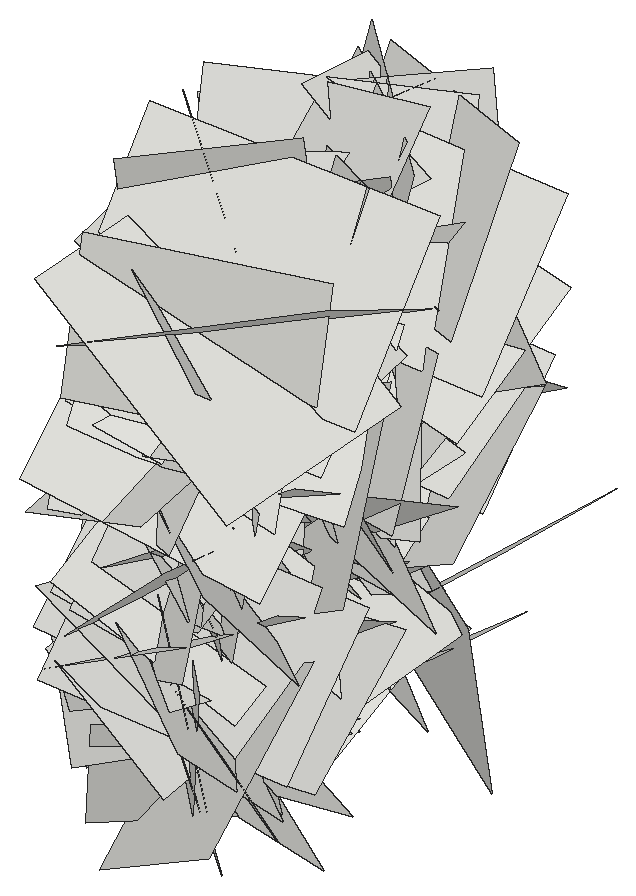
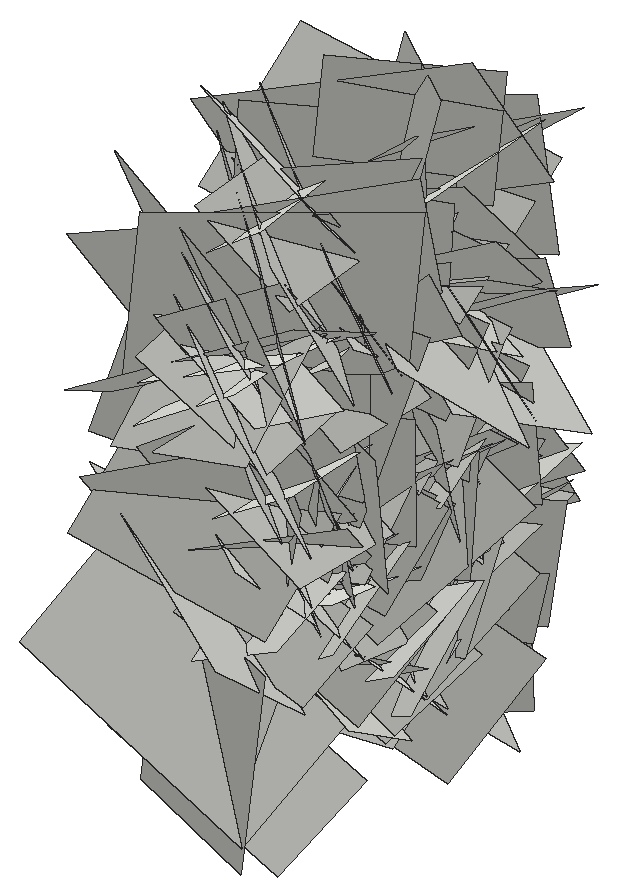
# SketchUp Ruby script. Lengths in inches.
U = 1.inch
M = Sketchup.active_model
def pt(a) = Geom::Point3d.new(a.map { |v| v * U })
def face(e, loops, mat)
  f = e.add_face(loops[0].map { |a| pt(a) })
  loops[1..].each { |l| e.add_face(l.map { |a| pt(a) }).erase! }
  f.material = f.back_material = mat if mat
  f
end
# faces: each face lists its corners as indices into pts; further lists are holes
def faces(e, pts, list, mat = nil) = list.each { |f| face(e, (f[0].is_a?(Array) ? f : [f]).map { |l| l.map { |i| pts[i] } }, mat) }
# xy, xz, yz: faces in a plane at the given z, y or x. An outline is a flat list of corners, or four numbers for a rectangle; further outlines are holes
def ring(l) = l.size == 4 ? [[l[0], l[1]], [l[2], l[1]], [l[2], l[3]], [l[0], l[3]]] : l.each_slice(2).to_a
def flat(e, list, mat, &to3) = list.each { |f| face(e, (f[0].is_a?(Array) ? f : [f]).map { |l| ring(l).map { |u, v| to3.(u, v) } }, mat) }
def xy(e, z, list, mat = nil) = flat(e, list, mat) { |x, y| [x, y, z] }
def xz(e, y, list, mat = nil) = flat(e, list, mat) { |x, z| [x, y, z] }
def yz(e, x, list, mat = nil) = flat(e, list, mat) { |y, z| [x, y, z] }
def lines(e, pts, list) = list.each { |a, b| e.add_line(pt(pts[a]), pt(pts[b])) }
# prism: a flat outline (further loops are holes) pulled along v
def prism(e, loops, v, mat = nil)
  f = face(e, loops, mat); d = Geom::Vector3d.new(v.map { |x| x * U })
  f.pushpull(f.normal.samedirection?(d) ? d.length : -d.length)
end
def box(e, o, s, mat = nil) = prism(e, [[o, [o[0] + s[0], o[1], o[2]], [o[0] + s[0], o[1] + s[1], o[2]], [o[0], o[1] + s[1], o[2]]]], [0, 0, s[2]], mat)
def at(x, y, z, deg = 0) = Geom::Transformation.translation(pt([x, y, z])) * Geom::Transformation.rotation(ORIGIN, Z_AXIS, deg.degrees)
def axes(o, x, y, z) = Geom::Transformation.new([*x, 0, *y, 0, *z, 0, *pt(o).to_a, 1])
def part(name) = M.definitions.add(name)
# library, detail: a bought-in or finely detailed component or shape, given as its bounding box
def library(name, o, s) = part(name).tap { |d| box(d.entities, o, s) }
def detail(e, o, s) = box(e.add_group.entities, o, s)
def put(e, d, t, mat = nil) = e.add_instance(d, t).tap { |i| i.material = mat if mat }
def group(e, t, mat = nil) = e.add_group.tap { |g| g.transformation = t; g.material = mat if mat }.entities
root = M.entities
c1 = part("Component\#6")
p = [[0.01,0,0],[0,3.24,4.54],[4.32,3.24,4.54],[4.33,0,0]]
faces(c1.entities,p,[[0,1,2,3]])
put(root,c1,axes([420.52,168.24,29.62],[-0.00844,-0.1319,-0.59476],[-0.00779,-0.59475,0.132],[0.64572,-0.0089,-0.00618]))
put(root,c1,axes([420.52,163.79,31.02],[-0.0186,-0.39942,0.51021],[-0.04828,0.50989,0.39761],[0.68514,0.02509,0.04187]))
put(root,c1,axes([420.52,167.3,30.05],[-0.09755,-0.36279,0.79394],[-0.2327,0.7823,0.33203],[0.89554,0.16375,0.17276]))
put(root,c1,axes([420.52,166.74,28.03],[-0.20581,0.5378,0.53941],[0.0447,0.5634,-0.54654],[0.80617,0.10606,0.16802]))
put(root,c1,axes([420.52,165.16,26.22],[0.00662,-0.41647,0.48084],[-0.04981,0.47925,0.41571],[0.67246,0.0396,0.02606]))
put(root,c1,axes([424.49,162.15,25.43],[0.09766,0.84172,-0.54191],[-0.18116,-0.52299,-0.84139],[-1.04557,0.16923,0.09516]))
put(root,c1,axes([420.52,170.38,37.22],[-0.01844,-0.65259,0.06973],[-0.0154,0.07012,0.65262],[0.69551,-0.01575,0.0163]))
put(root,c1,axes([424.49,159.15,32.85],[0.28722,0.93511,0.86971],[0.00467,0.88838,-0.95656],[-1.35365,0.20148,0.18123]))
put(root,c1,axes([420.52,168.23,31.98],[-0.11552,-0.73847,0.10601],[0.00435,0.10653,0.74638],[0.79079,-0.10846,0.01138]))
put(root,c1,axes([420.52,162.33,29.83],[-0.22776,0.38392,-0.75072],[0.01782,-0.77261,-0.39993],[0.89361,0.11326,-0.18337]))
put(root,c1,axes([424.49,165.04,27.71],[0.04822,0.07219,0.94774],[-0.14201,0.93984,-0.06516],[-0.99746,-0.13032,0.05509]))
put(root,c1,axes([420.52,171.91,32.4],[0.07209,-0.36069,-0.54144],[-0.07785,-0.54516,0.35394],[0.6852,-0.024,0.09718]))
put(root,c1,axes([424.49,167.29,35.58],[-0.17595,-0.29467,-0.74084],[-0.05215,-0.7515,0.30993],[-0.84352,0.10793,0.13537]))
put(root,c1,axes([424.49,157.3125,32.29],[0.25179,1.05256,0.51222],[-0.06429,0.53303,-1.06718],[-1.23914,0.18623,0.15945]))
put(root,c1,axes([420.52,168.82,35.84],[0.04533,0.37689,0.51175],[-0.01637,0.51337,-0.3768],[0.67349,-0.01289,-0.04361]))
put(root,c1,axes([420.52,159.46,22.85],[-0.09982,-0.0635,0.89488],[-0.1784,0.88507,0.04509],[0.93408,0.16225,0.10424]))
put(root,c1,axes([420.52,160.06,22.6],[-0.02839,-0.24478,0.77995],[-0.15528,0.76918,0.23637],[0.85248,0.13195,0.06903]))
put(root,c1,axes([420.52,159.67,28.14],[-0.12868,0.67272,0.52517],[-0.08613,0.51893,-0.68352],[0.90053,0.14576,0.00967]))
put(root,c1,axes([424.49,167.34,31.77],[0.2501,0.51374,1.1242],[0.05799,1.13903,-0.532],[-1.3089,0.14863,0.19123]))
put(root,c1,axes([420.52,158.39,26.84],[-0.02686,0.84806,0.10272],[-0.17857,0.09579,-0.83237],[0.88773,0.04493,-0.16432]))
put(root,c1,axes([420.52,169.17,27.35],[0.00515,-0.4485,-0.48712],[0.04455,-0.48594,0.44784],[0.70046,0.0342,-0.02491]))
put(root,c1,axes([424.49,161.79,25.53],[-0.01152,-0.82607,0.19056],[-0.15176,0.18963,0.81386],[-0.88572,-0.02175,-0.14193]))
put(root,c1,axes([424.49,164.2,31.01],[0.06613,-0.18181,-0.96198],[-0.02897,-0.96387,0.1804],[-1.03734,0.01533,-0.06637]))
put(root,c1,axes([420.52,169.92,30.86],[0.08798,0.07784,-0.70174],[-0.08853,-0.70052,-0.08758],[0.74315,-0.09267,0.07264]))
put(root,c1,axes([424.49,162.32,28.44],[-0.12821,-0.42216,-0.69512],[0.01339,-0.70366,0.42514],[-0.86197,0.05186,0.11]))
put(root,c1,axes([424.49,166.33,22.3],[0.05809,-0.87115,0.26873],[-0.09257,0.26296,0.87026],[-0.96191,-0.07791,-0.06752]))
put(root,c1,axes([424.49,171.77,39.47],[0.25632,-0.1505,-1.28885],[0.2021,-1.29268,0.18672],[-1.36053,-0.22038,-0.21508]))
put(root,c1,axes([420.52,167.69,34.89],[0.01272,-0.59445,-0.3878],[0.01652,-0.38754,0.59453],[0.75216,0.01856,-0.0065]))
put(root,c1,axes([420.52,168.18,25.35],[0.0356,-0.79141,-0.13903],[-0.13499,-0.14264,0.78117],[0.84098,0.01061,0.13127]))
put(root,c1,axes([424.49,163.85,33.45],[0.03445,-0.73428,-0.4148],[-0.17499,-0.41262,0.71747],[-0.87664,0.05351,-0.15952]))
put(root,c1,axes([424.49,158.45,30.92],[0.16236,0.46297,0.88251],[-0.09478,0.89566,-0.45434],[-1.05211,-0.00924,0.17712]))
put(root,c1,axes([424.49,166.53,31.68],[0.02185,0.89564,-0.0065],[-0.05171,-0.00537,-0.89456],[-0.948,0.02094,0.04865]))
put(root,c1,axes([424.49,171.21,38.93],[0.24063,-0.51313,-1.11059],[0.16085,-1.10901,0.54342],[-1.28679,-0.23458,-0.13976]))
put(root,c1,axes([420.52,171.89,34.33],[-0.10287,-0.74562,-0.1631],[0.15609,-0.17961,0.73351],[0.79385,-0.06131,-0.16536]))
put(root,c1,axes([424.49,162.43,26.35],[-0.02315,-0.70596,0.51236],[0.01203,0.51225,0.70629],[-0.92456,0.02434,-0.00364]))
put(root,c1,axes([424.49,162.61,28.57],[0.04222,-0.49534,0.62953],[-0.20196,0.60636,0.48917],[-0.82474,-0.17384,-0.08755]))
put(root,c1,axes([424.49,162.92,24.26],[-0.16568,0.16434,-0.80239],[0.1251,-0.80382,-0.18763],[-0.85913,-0.14874,0.12742]))
put(root,c1,axes([424.49,164.5,23.79],[-0.04443,0.667,0.37408],[-0.11412,0.36576,-0.66423],[-0.80255,-0.08894,0.07374]))
put(root,c1,axes([424.49,168.875,35.8],[-0.07444,0.7996,-0.0855],[-0.00091,-0.0859,-0.80263],[-0.85241,-0.06974,0.00832]))
put(root,c1,axes([420.52,164.96,33.58],[0.03363,-0.67551,-0.53197],[-0.14584,-0.52946,0.66412],[0.89967,-0.06058,0.12754]))
put(root,c1,axes([420.52,169.82,24.93],[0.00586,-0.68753,0.27068],[0.05817,0.27032,0.6855],[0.78107,-0.01497,-0.05308]))
put(root,c1,axes([424.49,164.8,26.41],[-0.06555,-0.88967,-0.10275],[0.1194,-0.1099,0.88381],[-0.94178,0.04799,0.1192]))
put(root,c1,axes([424.49,163.99,40.83],[-0.08038,0.23372,-0.81219],[0.10222,-0.80774,-0.24144],[-0.89001,-0.11388,0.04562]))
put(root,c1,axes([424.49,167.51,23.32],[0.04127,-0.8056,0.43064],[0.05085,0.43224,0.80425],[-0.96695,-0.01165,0.06068]))
put(root,c1,axes([424.49,164.95,29.96],[0.04265,0.57286,-0.52342],[-0.15347,-0.50938,-0.56862],[-0.80809,0.12697,0.08036]))
put(root,c1,axes([420.52,164.95,29.96],[-0.04265,0.57286,-0.52342],[0.15347,-0.50938,-0.56862],[0.80809,0.12697,0.08036]))
put(root,c1,axes([420.52,167.51,23.32],[-0.04127,-0.8056,0.43064],[-0.05085,0.43224,0.80425],[0.96695,-0.01165,0.06068]))
put(root,c1,axes([420.52,163.99,40.83],[0.08038,0.23372,-0.81219],[-0.10222,-0.80774,-0.24144],[0.89001,-0.11388,0.04562]))
put(root,c1,axes([420.52,164.8,26.41],[0.06555,-0.88967,-0.10275],[-0.1194,-0.1099,0.88381],[0.94178,0.04799,0.1192]))
put(root,c1,axes([424.49,169.82,24.93],[-0.00586,-0.68753,0.27068],[-0.05817,0.27032,0.6855],[-0.78107,-0.01497,-0.05308]))
put(root,c1,axes([424.49,164.96,33.58],[-0.03363,-0.67551,-0.53197],[0.14584,-0.52946,0.66412],[-0.89967,-0.06058,0.12754]))
put(root,c1,axes([420.52,168.875,35.8],[0.07444,0.7996,-0.0855],[0.00091,-0.0859,-0.80263],[0.85241,-0.06974,0.00832]))
put(root,c1,axes([420.52,164.5,23.79],[0.04443,0.667,0.37408],[0.11412,0.36576,-0.66423],[0.80255,-0.08894,0.07374]))
put(root,c1,axes([420.52,162.92,24.26],[0.16568,0.16434,-0.80239],[-0.1251,-0.80382,-0.18763],[0.85913,-0.14874,0.12742]))
put(root,c1,axes([420.52,162.61,28.57],[-0.04222,-0.49534,0.62953],[0.20196,0.60636,0.48917],[0.82474,-0.17384,-0.08755]))
put(root,c1,axes([420.52,162.43,26.35],[0.02315,-0.70596,0.51236],[-0.01203,0.51225,0.70629],[0.92456,0.02434,-0.00364]))
put(root,c1,axes([424.49,171.89,34.33],[0.10287,-0.74562,-0.1631],[-0.15609,-0.17961,0.73351],[-0.79385,-0.06131,-0.16536]))
put(root,c1,axes([420.52,171.21,38.93],[-0.24063,-0.51313,-1.11059],[-0.16085,-1.10901,0.54342],[1.28679,-0.23458,-0.13976]))
put(root,c1,axes([420.52,166.53,31.68],[-0.02185,0.89564,-0.0065],[0.05171,-0.00537,-0.89456],[0.948,0.02094,0.04865]))
put(root,c1,axes([420.52,158.45,30.92],[-0.16236,0.46297,0.88251],[0.09478,0.89566,-0.45434],[1.05211,-0.00924,0.17712]))
put(root,c1,axes([420.52,163.85,33.45],[-0.03445,-0.73428,-0.4148],[0.17499,-0.41262,0.71747],[0.87664,0.05351,-0.15952]))
put(root,c1,axes([424.49,168.18,25.35],[-0.0356,-0.79141,-0.13903],[0.13499,-0.14264,0.78117],[-0.84098,0.01061,0.13127]))
put(root,c1,axes([424.49,167.69,34.89],[-0.01272,-0.59445,-0.3878],[-0.01652,-0.38754,0.59453],[-0.75216,0.01856,-0.0065]))
put(root,c1,axes([420.52,171.77,39.47],[-0.25632,-0.1505,-1.28885],[-0.2021,-1.29268,0.18672],[1.36053,-0.22038,-0.21508]))
put(root,c1,axes([420.52,166.33,22.3],[-0.05809,-0.87115,0.26873],[0.09257,0.26296,0.87026],[0.96191,-0.07791,-0.06752]))
put(root,c1,axes([420.52,162.32,28.44],[0.12821,-0.42216,-0.69512],[-0.01339,-0.70366,0.42514],[0.86197,0.05186,0.11]))
put(root,c1,axes([424.49,169.92,30.86],[-0.08798,0.07784,-0.70174],[0.08853,-0.70052,-0.08758],[-0.74315,-0.09267,0.07264]))
put(root,c1,axes([420.52,164.2,31.01],[-0.06613,-0.18181,-0.96198],[0.02897,-0.96387,0.1804],[1.03734,0.01533,-0.06637]))
put(root,c1,axes([420.52,161.79,25.53],[0.01152,-0.82607,0.19056],[0.15176,0.18963,0.81386],[0.88572,-0.02175,-0.14193]))
put(root,c1,axes([424.49,169.17,27.35],[-0.00515,-0.4485,-0.48712],[-0.04455,-0.48594,0.44784],[-0.70046,0.0342,-0.02491]))
put(root,c1,axes([424.49,158.39,26.84],[0.02686,0.84806,0.10272],[0.17857,0.09579,-0.83237],[-0.88773,0.04493,-0.16432]))
put(root,c1,axes([424.49,159.67,28.14],[0.12868,0.67272,0.52517],[0.08613,0.51893,-0.68352],[-0.90053,0.14576,0.00967]))
put(root,c1,axes([424.49,160.06,22.6],[0.02839,-0.24478,0.77995],[0.15528,0.76918,0.23637],[-0.85248,0.13195,0.06903]))
put(root,c1,axes([424.49,159.46,22.85],[0.09982,-0.0635,0.89488],[0.1784,0.88507,0.04509],[-0.93408,0.16225,0.10424]))
put(root,c1,axes([424.49,168.82,35.84],[-0.04533,0.37689,0.51175],[0.01637,0.51337,-0.3768],[-0.67349,-0.01289,-0.04361]))
put(root,c1,axes([420.52,157.3125,32.29],[-0.25179,1.05256,0.51222],[0.06429,0.53303,-1.06718],[1.23914,0.18623,0.15945]))
put(root,c1,axes([420.52,167.29,35.58],[0.17595,-0.29467,-0.74084],[0.05215,-0.7515,0.30993],[0.84352,0.10793,0.13537]))
put(root,c1,axes([424.49,171.91,32.4],[-0.07209,-0.36069,-0.54144],[0.07785,-0.54516,0.35394],[-0.6852,-0.024,0.09718]))
put(root,c1,axes([420.52,165.04,27.71],[-0.04822,0.07219,0.94774],[0.14201,0.93984,-0.06516],[0.99746,-0.13032,0.05509]))
put(root,c1,axes([424.49,162.33,29.83],[0.22776,0.38392,-0.75072],[-0.01782,-0.77261,-0.39993],[-0.89361,0.11326,-0.18337]))
put(root,c1,axes([424.49,168.23,31.98],[0.11552,-0.73847,0.10601],[-0.00435,0.10653,0.74638],[-0.79079,-0.10846,0.01138]))
put(root,c1,axes([424.49,158.35,30.49],[0.08461,0.81055,-0.03501],[0.12527,-0.04642,-0.80528],[-0.85081,0.07377,-0.12204]))
put(root,c1,axes([420.52,159.15,32.85],[-0.28722,0.93511,0.86971],[-0.00467,0.88838,-0.95656],[1.35365,0.20148,0.18123]))
put(root,c1,axes([424.49,170.38,37.22],[0.01844,-0.65259,0.06973],[0.0154,0.07012,0.65262],[-0.69551,-0.01575,0.0163]))
put(root,c1,axes([420.52,162.15,25.43],[-0.09766,0.84172,-0.54191],[0.18116,-0.52299,-0.84139],[1.04557,0.16923,0.09516]))
put(root,c1,axes([424.49,165.16,26.22],[-0.00662,-0.41647,0.48084],[0.04981,0.47925,0.41571],[-0.67246,0.0396,0.02606]))
put(root,c1,axes([424.49,166.74,28.03],[0.20581,0.5378,0.53941],[-0.0447,0.5634,-0.54654],[-0.80617,0.10606,0.16802]))
put(root,c1,axes([424.49,167.3,30.05],[0.09755,-0.36279,0.79394],[0.2327,0.7823,0.33203],[-0.89554,0.16375,0.17276]))
put(root,c1,axes([424.49,163.79,31.02],[0.0186,-0.39942,0.51021],[0.04828,0.50989,0.39761],[-0.68514,0.02509,0.04187]))
put(root,c1,axes([424.49,168.24,29.62],[0.00844,-0.1319,-0.59476],[0.00779,-0.59475,0.132],[-0.64572,-0.0089,-0.00618]))
put(root,c1,axes([420.52,168.37,37.02],[-0.06582,-0.55881,-0.84289],[0.17414,-0.83883,0.54402],[1.05774,0.10333,-0.14201]))
put(root,c1,axes([420.52,162.55,24.47],[0.08094,0.6993,-0.63815],[0.06519,-0.64254,-0.69674],[1.00139,-0.01469,0.09694]))
put(root,c1,axes([424.49,167.47,38.84],[0.19203,-0.25676,-0.78485],[0.09527,-0.79261,0.28005],[-0.87013,-0.14344,-0.14255]))
put(root,c1,axes([424.49,168.14,25.37],[0.00005,-0.54267,0.44601],[0.16088,0.43548,0.52984],[-0.72699,0.09633,0.11728]))
put(root,c1,axes([420.52,169.13,31.47],[0.22896,-0.22184,-0.76377],[0.12794,-0.77313,0.25869],[0.83329,0.17965,0.17014]))
put(root,c1,axes([420.52,164.67,22.86],[-0.07455,-1.03669,0.46758],[0.01691,0.46753,1.03897],[1.20537,-0.07068,0.01434]))
put(root,c1,axes([424.49,161.42,33.85],[0.12931,-0.58697,0.4315],[0.06321,0.44408,0.58723],[-0.76963,-0.06214,0.12073]))
put(root,c1,axes([420.52,160.7,27.63],[-0.09928,0.64406,-0.88513],[0.13228,-0.87629,-0.65083],[1.15276,0.15602,-0.00154]))
put(root,c1,axes([420.52,159.57,38.3125],[-0.19748,1.37219,0.09956],[-0.15298,0.08042,-1.37849],[1.4503,0.19533,-0.13185]))
put(root,c1,axes([424.49,165.91,24.52],[-0.03596,-0.58924,0.24858],[0.15481,0.23521,0.57749],[-0.65999,0.08727,0.12191]))
put(root,c1,axes([420.52,166.55,31.56],[0.0814,0.41102,-0.8284],[0.17089,-0.82447,-0.39413],[0.96524,0.11131,0.13964]))
put(root,c1,axes([424.49,169.1,21.1],[0.05323,-0.42134,0.48328],[0.06346,0.48572,0.41725],[-0.67666,0.01241,0.07715]))
put(root,c1,axes([420.52,166.67,25.47],[-0.29316,-1.18227,0.54308],[0.10516,0.53443,1.21398],[1.37509,-0.29293,0.02294]))
put(root,c1,axes([420.52,168.75,37.98],[-0.06882,-0.53698,-1.12739],[-0.1022,-1.12338,0.54063],[1.31971,-0.115,-0.01692]))
put(root,c1,axes([420.52,158.58,28.72],[0.17742,0.80309,0.64454],[-0.10421,0.66248,-0.79991],[1.08655,-0.0676,-0.18196]))
put(root,c1,axes([424.49,163.1,21.29],[0.03251,-0.459,0.52355],[0.17075,0.51451,0.44164],[-0.71801,0.10157,0.12873]))
put(root,c1,axes([420.52,169.04,36.23],[-0.04162,0.78981,-0.64322],[0.24351,-0.62024,-0.77563],[1.05189,0.17484,0.15411]))
put(root,c1,axes([420.52,170.89,20.28],[0.12274,-1.02279,0.17958],[-0.0333,0.17716,1.02926],[1.10024,0.11946,0.01112]))
put(root,c1,axes([420.52,167.53,29.6],[0.04916,0.6172,0.8297],[0.08211,0.82613,-0.61887],[1.09305,-0.08981,0.00917]))
put(root,c1,axes([420.52,171.44,27.64],[0.05126,-0.8571,0.56567],[0.11133,0.56746,0.85083],[1.08285,-0.01777,-0.11425]))
put(root,c1,axes([424.49,163.13,28.77],[0.13219,-0.55975,0.33448],[0.05965,0.34851,0.56225],[-0.68862,-0.07726,0.11291]))
put(root,c1,axes([420.52,163.625,35.04],[0.27654,-0.44632,0.88094],[-0.09901,0.89592,0.48157],[1.04211,0.20356,-0.18801]))
put(root,c1,axes([420.52,167.41,29.34],[-0.20833,-0.42173,1.22713],[0.0869,1.23461,0.43743],[1.37269,-0.14217,0.15855]))
put(root,c1,axes([420.52,168.84,39.14],[0.0295,-0.69575,-0.73723],[0.22295,-0.71749,0.68506],[1.05113,0.17171,-0.12461]))
put(root,c1,axes([420.52,163.85,26.9],[0.03329,1.04875,0.11229],[0.24045,0.10299,-1.02538],[1.09187,-0.05466,0.22238]))
put(root,c1,axes([420.52,160.22,28.4],[0.15479,0.80897,-0.76348],[-0.02106,-0.76802,-0.81757],[1.17891,-0.11994,0.08565]))
put(root,c1,axes([420.52,169.63,32.59],[0.01533,-0.4611,-1.03377],[0.17767,-1.02158,0.45801],[1.18663,0.15892,-0.05522]))
put(root,c1,axes([420.52,159.8,34.2],[-0.03301,0.77795,0.85676],[0.24326,0.8442,-0.75821],[1.20233,-0.14944,0.17692]))
put(root,c1,axes([420.52,166.97,25.06],[-0.03339,-0.82276,-0.77538],[0.30966,-0.75526,0.78954],[1.15769,0.17829,-0.23355]))
put(root,c1,axes([420.52,165.55,34.43],[-0.04885,1.13911,0.54464],[0.08516,0.54654,-1.13629],[1.33566,0.00681,0.09237]))
put(root,c1,axes([420.52,164.92,23.28],[0.02573,-1.02703,-0.88101],[-0.12942,-0.87922,1.02158],[1.42847,-0.06116,0.10843]))
put(root,c1,axes([420.52,160.96,32.62],[0.12215,0.75895,-0.88724],[0.014,-0.89234,-0.7616],[1.23753,-0.06482,0.09619]))
put(root,c1,axes([420.52,172.54,38.57],[-0.12011,-0.4932,-1.18141],[0.20578,-1.17893,0.47355],[1.34134,0.1367,-0.17844]))
put(root,c1,axes([420.52,171.44,26.6],[-0.03428,0.27698,-1.26013],[0.06702,-1.25867,-0.27828],[1.36598,0.0687,-0.01797]))
put(root,c1,axes([420.52,173.53,27.66],[0.08068,-0.97468,-0.75893],[0.01331,-0.75972,0.97695],[1.30935,0.06778,0.03684]))
put(root,c1,axes([420.52,158.99,33.95],[0.09747,0.08794,1.12692],[0.17247,1.11783,-0.1005],[1.18568,-0.16983,-0.07802]))
put(root,c1,axes([420.52,166.62,31.96],[0.21061,0.75098,-0.921],[-0.02022,-0.93165,-0.76377],[1.25951,-0.14053,0.14175]))
put(root,c1,axes([420.52,158.06,26.05],[0.19995,0.52409,1.06255],[0.00833,1.07535,-0.5318],[1.25583,-0.09057,-0.16565]))
put(root,c1,axes([420.52,172.42,21.79],[0.22827,-1.35966,0.24048],[-0.1567,0.21929,1.3722],[1.45519,0.2369,0.11004]))
put(root,c1,axes([420.52,165.11,34.6875],[0.03998,0.77126,1.05992],[0.2457,1.03973,-0.76482],[1.36759,-0.20934,0.10642]))
put(root,c1,axes([420.52,159.18,36.25],[0.04304,0.74935,1.15311],[0.14712,1.14549,-0.74928],[1.45028,-0.13844,0.04179]))
put(root,c1,axes([420.52,168.45,29.92],[0.2904,-0.81126,-1.09363],[-0.15157,-1.12651,0.79984],[1.4354,0.04517,0.30571]))
put(root,c1,axes([420.52,157.9,37.93],[0.24747,1.3445,0.30187],[-0.11522,0.32319,-1.35538],[1.4561,-0.20293,-0.15855]))
put(root,c1,axes([420.52,163.2,33.68],[0.16473,-1.2102,0.57798],[0.2383,0.59712,1.18983],[1.40149,0.04071,-0.27024]))
